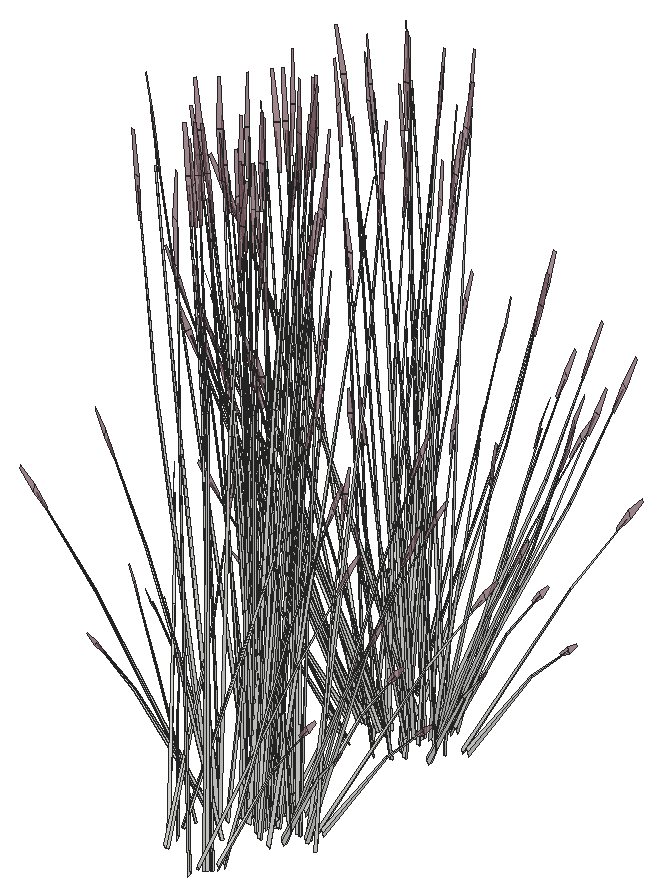
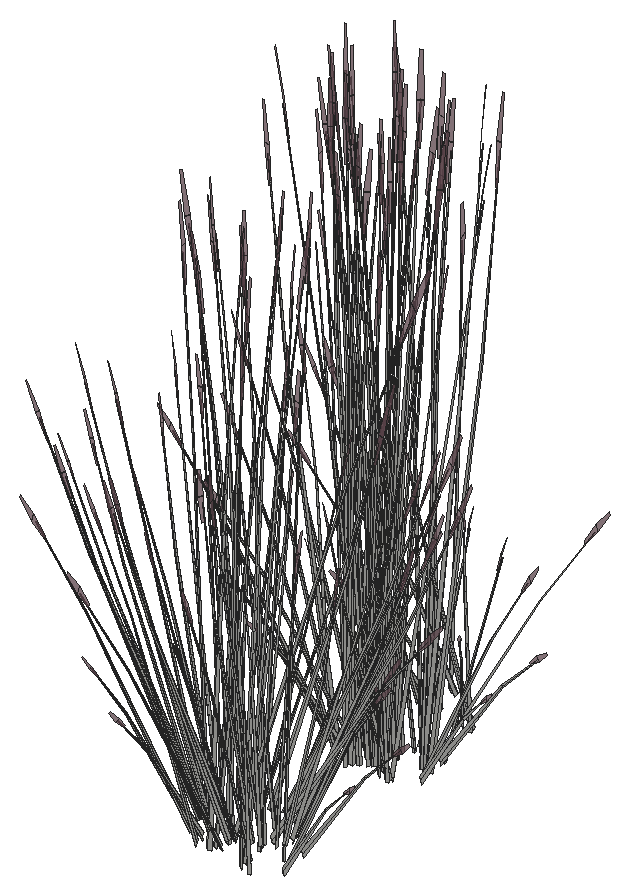
# SketchUp Ruby script. Lengths in inches.
U = 1.inch
M = Sketchup.active_model
def pt(a) = Geom::Point3d.new(a.map { |v| v * U })
def face(e, loops, mat)
  f = e.add_face(loops[0].map { |a| pt(a) })
  loops[1..].each { |l| e.add_face(l.map { |a| pt(a) }).erase! }
  f.material = f.back_material = mat if mat
  f
end
# faces: each face lists its corners as indices into pts; further lists are holes
def faces(e, pts, list, mat = nil) = list.each { |f| face(e, (f[0].is_a?(Array) ? f : [f]).map { |l| l.map { |i| pts[i] } }, mat) }
# xy, xz, yz: faces in a plane at the given z, y or x. An outline is a flat list of corners, or four numbers for a rectangle; further outlines are holes
def ring(l) = l.size == 4 ? [[l[0], l[1]], [l[2], l[1]], [l[2], l[3]], [l[0], l[3]]] : l.each_slice(2).to_a
def flat(e, list, mat, &to3) = list.each { |f| face(e, (f[0].is_a?(Array) ? f : [f]).map { |l| ring(l).map { |u, v| to3.(u, v) } }, mat) }
def xy(e, z, list, mat = nil) = flat(e, list, mat) { |x, y| [x, y, z] }
def xz(e, y, list, mat = nil) = flat(e, list, mat) { |x, z| [x, y, z] }
def yz(e, x, list, mat = nil) = flat(e, list, mat) { |y, z| [x, y, z] }
def lines(e, pts, list) = list.each { |a, b| e.add_line(pt(pts[a]), pt(pts[b])) }
# prism: a flat outline (further loops are holes) pulled along v
def prism(e, loops, v, mat = nil)
  f = face(e, loops, mat); d = Geom::Vector3d.new(v.map { |x| x * U })
  f.pushpull(f.normal.samedirection?(d) ? d.length : -d.length)
end
def box(e, o, s, mat = nil) = prism(e, [[o, [o[0] + s[0], o[1], o[2]], [o[0] + s[0], o[1] + s[1], o[2]], [o[0], o[1] + s[1], o[2]]]], [0, 0, s[2]], mat)
def at(x, y, z, deg = 0) = Geom::Transformation.translation(pt([x, y, z])) * Geom::Transformation.rotation(ORIGIN, Z_AXIS, deg.degrees)
def axes(o, x, y, z) = Geom::Transformation.new([*x, 0, *y, 0, *z, 0, *pt(o).to_a, 1])
def part(name) = M.definitions.add(name)
# library, detail: a bought-in or finely detailed component or shape, given as its bounding box
def library(name, o, s) = part(name).tap { |d| box(d.entities, o, s) }
def detail(e, o, s) = box(e.add_group.entities, o, s)
def put(e, d, t, mat = nil) = e.add_instance(d, t).tap { |i| i.material = mat if mat }
def group(e, t, mat = nil) = e.add_group.tap { |g| g.transformation = t; g.material = mat if mat }.entities
root = M.entities
M.materials.add("LightPink_Translucent").color = [144, 107, 117]
M.materials["LightPink_Translucent"].alpha = 0.75
c1 = part("blade")
p = [[2.15,0.21,22],[0,0.17,0],[0.09,0.45,0],[2.18,0.31,22],[2.29,0.31,22],[0.38,0.45,0],
  [2.48,0.24,33],[2.49,0.24,33],[2.48,0.22,33]]
faces(c1.entities,p,[[0,1,2,3],[4,5,2,3],[6,3,4,7],[8,0,3,6]])
c2 = part("seeds")
p = [[0.3,-0.1,1.38],[-0.01,-0.03,1.59],[-0.01,-0.03,0.03],[0.14,-0.07,-0.07],[0.29,-0.03,3],[0.15,0.01,3.11]]
faces(c2.entities,p,[[0,1,2,3],[1,0,4,5]],"LightPink_Translucent")
c3 = part("blade with seeds")
put(c3.entities,c1,at(0,0,0))
put(c3.entities,c2,axes([2.4,0.25,30.99],[1.5799,-0.05474,1.17369],[-0.12525,1.92788,0.29478],[-0.07173,-0.02425,1.56792]))
put(root,c3,axes([273.84,375.7,124.88],[1.11998,0.21207,0.30756],[-0.2802,0.75803,-0.36492],[-0.18537,0.09487,1.64885]))
put(root,c3,axes([275.27,375.64,125.3125],[-0.5037,-0.18761,1.1486],[0.6504,-0.19062,0.84392],[0.17543,0.16147,0.25299]))
put(root,c3,axes([274.52,376.11,124.92],[0.55932,0.6538,0],[-0.93577,0.36461,-0.51607],[-0.21313,0.08304,1.63711]))
put(root,c3,axes([274.04,373.52,125.39],[-0.02444,-0.61432,1.41272],[1.10603,0.15924,0.59816],[-0.26159,0.33615,1.3335]))
put(root,c3,axes([270.82,381.5,124.95],[-0.55932,-0.6538,0],[0.93577,-0.36461,-0.51607],[0.21313,-0.08304,1.63711]))
put(root,c3,axes([272.05,380.71,124.71],[-0.61821,0.37431,-0.03893],[-0.56645,-0.40995,-0.17649],[-0.03988,-0.11616,0.58215]))
put(root,c3,axes([275.35,376.49,125.22],[-0.57368,-0.02046,1.0506],[0.37886,-0.43461,0.58006],[0.22663,0.15441,0.8241]))
put(root,c3,axes([276.55,382.52,125.17],[-0.31959,-0.01933,1.43002],[-0.32741,-0.51843,-0.30754],[0.39262,-0.14666,0.61141]))
put(root,c3,axes([273.48,375.4375,125.14],[0.01579,-0.21629,1.43002],[0.75442,-0.24159,-0.30754],[0.23289,0.25887,0.61141]))
put(root,c3,axes([276.92,381.57,125.35],[-0.29798,0.33213,1.1486],[-0.25612,-0.44624,0.84392],[0.24611,-0.11182,0.25299]))
put(root,c3,axes([270.05,377.24,125.3125],[-0.02315,-0.38796,1.1486],[0.57853,0.27671,0.84392],[-0.11378,0.18492,0.25299]))
put(root,c3,axes([268.98,381.39,124.71],[-0.25807,0.53277,-0.03893],[-0.79428,-0.16389,-0.17649],[-0.1206,-0.08714,0.58215]))
put(root,c3,axes([269.57,376.4,125.37],[0.8127,-0.11554,0.06507],[0.18684,0.46549,-0.86304],[-0.05152,0.23564,0.7736]))
put(root,c3,axes([268.55,383.82,124.95],[-1.11865,0,0],[0,-0.72922,-0.51607],[0,-0.16609,1.63711]))
put(root,c3,axes([268.74,382.52,125.17],[0.17466,0.18165,1.43002],[-0.40248,0.49377,-0.30754],[-0.41327,-0.11802,0.61141]))
put(root,c3,axes([269.42,383.63,124.91],[-0.83213,0.54855,0.30756],[-0.83263,-0.54278,-0.36492],[-0.02906,-0.15578,1.64885]))
put(root,c3,axes([271.85,376.06,127.53],[0.42698,0.53052,-0.71045],[-0.87893,0.29566,0.08574],[0.09984,0.25633,1.00501]))
put(root,c3,axes([269.38,376.89,125.14],[0.28231,-0.10293,1.43002],[0.69701,0.31035,-0.30754],[-0.20746,0.26854,0.61141]))
put(root,c3,axes([272.0625,383.88,125.01],[1.00799,0.31623,0.24065],[-0.48511,0.65709,0.50002],[0,-0.15147,1.60543]))
put(root,c3,axes([267.7,383.0625,125.35],[0.57115,-0.04669,1.1486],[-0.36229,0.41137,0.84392],[-0.28224,-0.06171,0.25299]))
put(root,c3,axes([271.74,383.44,125.3],[-0.97146,0.04028,0.44739],[-0.08785,-0.66859,-0.21531],[0.17391,-0.06776,1.43643]))
put(root,c3,axes([269.23,383.93,125.06],[0,0.65246,0.49651],[-1.00089,0,0],[0,-0.1486,1.57504]))
put(root,c3,axes([274.94,381.66,124.96],[0.55932,-0.6538,0],[0.93577,0.36461,-0.51607],[0.21313,0.08304,1.63711]))
put(root,c3,axes([271.7,383.68,124.94],[0.38895,0.72959,0.45755],[-1.11135,0.2537,0.17955],[0.01358,-0.13406,1.58856]))
put(root,c3,axes([277.14,384.24,124.5625],[-0.57619,0.0783,1.41583],[-0.09171,-0.62326,0.08104],[0.40356,-0.09434,0.80566]))
put(root,c3,axes([278.19,383.69,124.84],[-0.55463,-0.41721,-0.06488],[0.60744,-0.38228,-0.29416],[0.17212,-0.02691,0.97024]))
put(root,c3,axes([271.51,384.26,125.3],[-0.43405,0.58792,0.44739],[-0.90188,-0.28295,-0.21531],[0,-0.13553,1.43643]))
put(root,c3,axes([273.1,383.75,124.79],[0,-0.75495,0],[1.11865,0,0],[0,0,1.79456]))
put(root,c3,axes([274.46,382,125.06],[-0.83726,-0.32623,0.49651],[0.50045,-0.58498,0],[0.19069,0.0743,1.57504]))
put(root,c3,axes([272.57,383.27,124.94],[-0.74176,0.59212,0.45755],[-0.88124,-0.52269,0.17955],[0.17882,-0.05909,1.58856]))
put(root,c3,axes([273.38,384.33,124.88],[-0.83213,-0.56158,-0.06131],[0.83263,-0.56193,0],[-0.02906,-0.01961,1.75571]))
put(root,c3,axes([271.29,382.3,125.05],[-0.25843,0.64844,0.17642],[-0.9457,-0.1835,0.35086],[0.16336,-0.00316,1.60407]))
put(root,c3,axes([273.26,383.02,125.2],[0.17258,-0.58229,0.1448],[0.84319,0.10108,-0.41347],[0.15345,0.05979,1.26744]))
put(root,c3,axes([271.8,384.4,124.94],[1.13071,0.13747,0.45755],[-0.23011,0.77639,0.17955],[-0.16524,-0.07497,1.58856]))
put(root,c3,axes([272.9,383.17,125.3],[-0.53742,-0.54764,0.44739],[0.81403,-0.38564,-0.21531],[0.17391,0.06776,1.43643]))
put(root,c3,axes([271.19,385.64,125.05],[0.96132,-0.17317,0.17642],[0.23737,0.64447,0.35086],[-0.08574,-0.0939,1.60407]))
put(root,c3,axes([273.86,383.92,124.79],[1.00089,0,0],[0,0.67548,0],[0,0,1.78407]))
put(root,c3,axes([274.15,382.33,125.05],[-0.96132,0.17317,0.17642],[-0.23737,-0.64447,0.35086],[0.08574,0.0939,1.60407]))
put(root,c3,axes([273.54,383.57,124.96],[-1.13071,-0.13747,0.49198],[0.23011,-0.77639,0.19306],[0.16524,0.07497,1.70813]))
put(root,c3,axes([272.64,385.49,124.78],[-0.29189,-0.56252,0],[0.83351,-0.19699,0],[0,0,1.54371]))
put(root,c3,axes([272.08,384.95,125.2],[-0.17258,0.58229,0.1448],[-0.84319,-0.10108,-0.41347],[-0.15345,-0.05979,1.26744]))
put(root,c3,axes([274.05,385.68,125.05],[0.25843,-0.64844,0.17642],[0.9457,0.1835,0.35086],[-0.16336,0.00316,1.60407]))
put(root,c3,axes([273.84,384.2,124.8],[0.62448,0.42144,0],[-0.62448,0.42144,0],[0,0,1.69266]))
put(root,c3,axes([275.53,384.02,125.05],[-0.70288,-0.47526,0.17642],[0.70832,-0.46097,0.35086],[-0.07763,0.09706,1.60407]))
put(root,c3,axes([278.34,384.46,125.35],[-0.55274,0.10771,1.1486],[0.26018,-0.44517,0.84392],[0.29323,0.03046,0.25299]))
put(root,c3,axes([272.43,385.74,124.78],[-0.90188,-0.29293,0],[0.43405,-0.60866,0],[0,0,1.62707]))
put(root,c3,axes([270.88,385.97,125.06],[0.83726,0.32623,0.49651],[-0.50045,0.58498,0],[-0.19069,-0.0743,1.57504]))
put(root,c3,axes([273.83,383.71,125.3],[0.43405,-0.58792,0.44739],[0.90188,0.28295,-0.21531],[0,0.13553,1.43643]))
put(root,c3,axes([273.67,384.05,124.87],[0,0.75458,-0.05637],[-1.11865,0,0],[0,0.02371,1.79368]))
put(root,c3,axes([270.4,386.31,124.95],[-0.55932,0.6538,0],[-0.93577,-0.36461,-0.51607],[-0.21313,-0.08304,1.63711]))
put(root,c3,axes([276.11,384.04,125.06],[0,-0.65246,0.49651],[1.00089,0,0],[0,0.1486,1.57504]))
put(root,c3,axes([273.6,384.53,125.3],[0.97146,-0.04028,0.44739],[0.08785,0.66859,-0.21531],[-0.17391,0.06776,1.43643]))
put(root,c3,axes([274.21,383.85,125.2],[0.83351,-0.19028,0.1448],[0.29189,0.54335,-0.41347],[0,0.11958,1.26744]))
put(root,c3,axes([277.31,385.17,125.17],[-0.21545,-0.16047,1.43002],[0.28033,-0.53085,-0.30754],[0.43591,0.07191,0.61141]))
put(root,c3,axes([273.45,385.75,124.78],[0.90188,0.29293,0],[-0.43405,0.60866,0],[0,0,1.74954]))
put(root,c3,axes([273.8125,386.4,124.77],[-0.55235,-0.65609,-0.05142],[0.93577,-0.36461,0.51607],[-0.23059,0.06247,1.6363]))
put(root,c3,axes([273.62,384.81,125.2],[0.66093,0.39201,0.1448],[-0.5513,0.44227,-0.41347],[-0.15345,0.05979,1.26744]))
put(root,c3,axes([274.32,386.02,125.06],[0.83726,-0.32623,0.49651],[0.50045,0.58498,0],[-0.19069,0.0743,1.57504]))
put(root,c3,axes([273.13,385.51,124.87],[0.38895,0.74956,-0.06012],[-1.11135,0.26265,0],[0.01358,0.02618,1.72173]))
put(root,c3,axes([267.54,385.17,125.17],[0.3109,0.05356,1.43002],[0.20038,0.54709,-0.30754],[-0.42231,0.10241,0.61141]))
put(root,c3,axes([276.79,384.15,124.96],[1.11865,0,0],[0,0.72922,-0.51607],[0,0.16609,1.63711]))
put(root,c3,axes([276.34,384.52,124.78],[-1.1181,-0.00522,-0.04976],[0,-0.72922,0.49943],[-0.03514,0.166,1.58352]))
put(root,c3,axes([266.89,386.3125,125.35],[0.37283,-0.29571,1.1486],[0.14711,0.46813,0.84392],[-0.26943,0.08382,0.25299]))
put(root,c3,axes([273.84,386.06,124.91],[1.11998,0.21207,0.30756],[-0.2802,0.75803,-0.36492],[-0.18537,0.09487,1.64885]))
put(root,c3,axes([275.27,386,125.35],[-0.5037,-0.18761,1.1486],[0.6504,-0.19062,0.84392],[0.17543,0.16147,0.25299]))
put(root,c3,axes([274.52,386.48,124.95],[0.55932,0.6538,0],[-0.93577,0.36461,-0.51607],[-0.21313,0.08304,1.63711]))
put(root,c3,axes([274.04,383.89,125.42],[-0.02444,-0.61432,1.41272],[1.10603,0.15924,0.59816],[-0.26159,0.33615,1.3335]))
put(root,c3,axes([275.35,386.85,125.25],[-0.57368,-0.02046,1.0506],[0.37886,-0.43461,0.58006],[0.22663,0.15441,0.8241]))
put(root,c3,axes([273.48,385.8,125.17],[0.01579,-0.21629,1.43002],[0.75442,-0.24159,-0.30754],[0.23289,0.25887,0.61141]))
put(root,c3,axes([270.05,387.6,125.35],[-0.02315,-0.38796,1.1486],[0.57853,0.27671,0.84392],[-0.11378,0.18492,0.25299]))
put(root,c3,axes([269.57,386.76,125.4],[0.8127,-0.11554,0.06507],[0.18684,0.46549,-0.86304],[-0.05152,0.23564,0.7736]))
put(root,c3,axes([269.38,387.26,125.17],[0.28231,-0.10293,1.43002],[0.69701,0.31035,-0.30754],[-0.20746,0.26854,0.61141]))
put(root,c3,axes([274.1,398.08,124.51],[-0.25429,0.13207,1.43002],[-0.76157,-0.23115,-0.30754],[0.14117,-0.28747,0.61141]))
put(root,c3,axes([272.94,398.54,126.9],[-0.42698,-0.53052,-0.71045],[0.87893,-0.29566,0.08574],[-0.09984,-0.25633,1.00501]))
put(root,c3,axes([270.16,397.83,124.51],[-0.05417,0.21344,1.43002],[-0.79196,0.17867,-0.30754],[-0.18512,-0.27588,0.61141]))
put(root,c3,axes([274.72,399.06,126.9],[0.02328,-0.60353,-0.71045],[0.98022,0.04053,0.08574],[0.10344,-0.25568,1.00501]))
put(root,c3,axes([273.02,398.09,126.44],[0.2697,-0.50175,-0.35414],[0.78684,0.14635,0.4572],[-0.07215,-0.20201,0.87481]))
put(root,c3,axes([272.62,398.43,126.6],[-0.87941,-0.16356,-0.51099],[0.30143,-0.56078,-0.3958],[-0.08064,-0.22578,0.97773]))
put(root,c3,axes([273.16,397.03,124.68],[0.11476,0.38047,1.1486],[-0.63664,-0.21072,0.84392],[0.06851,-0.19481,0.25299]))
put(root,c3,axes([274.52,398.86,126.6],[-0.64041,-0.4384,-0.51099],[0.67652,-0.38394,-0.3958],[0.09744,-0.22274,0.97773]))
put(root,c3,axes([275.12,398.69,126.44],[0.60531,-0.34352,-0.35414],[0.573,0.39225,0.4572],[0.08718,-0.19929,0.87481]))
put(root,c3,axes([269.89,397.48,124.68],[0.46666,0.22709,1.1486],[-0.67962,0.13651,0.84392],[-0.14541,-0.17452,0.25299]))
put(root,c3,axes([271.02,398.6875,126.9],[-0.76283,-0.31537,-0.71045],[0.54213,-0.55263,0.08574],[-0.27638,-0.1883,1.00501]))
put(root,c3,axes([270.75,398.27,126.44],[-0.13817,-0.52554,-0.35414],[0.78985,-0.13877,0.4572],[-0.21215,-0.1506,0.87481]))
put(root,c3,axes([270.66,398.7,126.6],[-0.88277,0.1551,-0.51099],[-0.15442,-0.58737,-0.3958],[-0.23711,-0.16832,0.97773]))
put(root,c3,axes([275.875,400.11,126.9],[0.4673,-0.51481,-0.71045],[0.81887,0.36587,0.08574],[0.27902,-0.18652,1.00501]))
put(root,c3,axes([275.85,399.87,126.6],[-0.22982,-0.59576,-0.51099],[0.87033,-0.10422,-0.3958],[0.24941,-0.16002,0.97773]))
put(root,c3,axes([272.84,402.26,125.24],[0.77308,0.2631,1.51261],[-0.75736,0.56681,0.59816],[-0.33924,-0.33594,1.26806]))
put(root,c3,axes([276.55,399.63,124.51],[-0.31959,-0.01933,1.43002],[-0.32741,-0.51843,-0.30754],[0.39262,-0.14666,0.61141]))
put(root,c3,axes([276.92,398.68,124.68],[-0.29798,0.33213,1.1486],[-0.25612,-0.44624,0.84392],[0.24611,-0.11182,0.25299]))
put(root,c3,axes([276.49,399.93,126.44],[0.77872,-0.09325,-0.35414],[0.20563,0.53305,0.4572],[0.22316,-0.14318,0.87481]))
put(root,c3,axes([268.92,399.2,126.44],[-0.50902,-0.40851,-0.35414],[0.58122,-0.38671,0.4572],[-0.29531,-0.05884,0.87481]))
put(root,c3,axes([269.46,399.47,126.9],[-0.89428,-0.01571,-0.71045],[0.06006,-0.66153,0.08574],[-0.37886,-0.06981,1.00501]))
put(root,c3,axes([269.17,399.6,126.6],[-0.6496,0.4322,-0.51099],[-0.5689,-0.45657,-0.3958],[-0.33005,-0.06576,0.97773]))
put(root,c3,axes([267.7,400.18,124.68],[0.57115,-0.04669,1.1486],[-0.36229,0.41137,0.84392],[-0.28224,-0.06171,0.25299]))
put(root,c3,axes([271.74,400.56,124.63],[-0.97146,0.04028,0.44739],[-0.08785,-0.66859,-0.21531],[0.17391,-0.06776,1.43643]))
put(root,c3,axes([269.23,401.04,124.39],[0,0.65246,0.49651],[-1.00089,0,0],[0,-0.1486,1.57504]))
put(root,c3,axes([276.26,401.1875,126.6],[0.24236,-0.59349,-0.51099],[0.83094,0.20343,-0.3958],[0.33455,-0.05442,0.97773]))
put(root,c3,axes([271.51,401.37,124.63],[-0.43405,0.58792,0.44739],[-0.90188,-0.28295,-0.21531],[0,-0.13553,1.43643]))
put(root,c3,axes([274.46,399.11,124.39],[-0.83726,-0.32623,0.49651],[0.50045,-0.58498,0],[0.19069,0.0743,1.57504]))
put(root,c3,axes([276.1,401.4,126.9],[0.78611,-0.28816,-0.71045],[0.4381,0.59317,0.08574],[0.37982,-0.06738,1.00501]))
put(root,c3,axes([271.29,399.41,124.39],[-0.25843,0.64844,0.17642],[-0.9457,-0.1835,0.35086],[0.16336,-0.00316,1.60407]))
put(root,c3,axes([272.9,400.28,124.63],[-0.53742,-0.54764,0.44739],[0.81403,-0.38564,-0.21531],[0.17391,0.06776,1.43643]))
put(root,c3,axes([271.19,402.75,124.39],[0.96132,-0.17317,0.17642],[0.23737,0.64447,0.35086],[-0.08574,-0.0939,1.60407]))
put(root,c3,axes([276.76,401.46,126.44],[0.74348,0.18202,-0.35414],[-0.21685,0.53102,0.4572],[0.29933,-0.04869,0.87481]))
put(root,c3,axes([268.03,400.61,126.44],[-0.74348,-0.18202,-0.35414],[0.21685,-0.53102,0.4572],[-0.29933,0.04869,0.87481]))
put(root,c3,axes([274.15,399.44,124.39],[-0.96132,0.17317,0.17642],[-0.23737,-0.64447,0.35086],[0.08574,0.0939,1.60407]))
put(root,c3,axes([274.05,402.79,124.39],[0.25843,-0.64844,0.17642],[0.9457,0.1835,0.35086],[-0.16336,0.00316,1.60407]))
put(root,c3,axes([270.29,400.53,125.26],[0.25429,-0.09438,1.77064],[0.08769,0.65901,0.13857],[-0.5508,0.08745,0.63284]))
put(root,c3,axes([275.53,401.13,124.39],[-0.70288,-0.47526,0.17642],[0.70832,-0.46097,0.35086],[-0.07763,0.09706,1.60407]))
put(root,c3,axes([278.34,401.57,124.68],[-0.55274,0.10771,1.1486],[0.26018,-0.44517,0.84392],[0.29323,0.03046,0.25299]))
put(root,c3,axes([270.88,403.08,124.39],[0.83726,0.32623,0.49651],[-0.50045,0.58498,0],[-0.19069,-0.0743,1.57504]))
put(root,c3,axes([273.83,400.82,124.63],[0.43405,-0.58792,0.44739],[0.90188,0.28295,-0.21531],[0,0.13553,1.43643]))
put(root,c3,axes([268.54,400.88,126.6],[-0.24236,0.59349,-0.51099],[-0.83094,-0.20343,-0.3958],[-0.33455,0.05442,0.97773]))
put(root,c3,axes([276.11,401.15,124.39],[0,-0.65246,0.49651],[1.00089,0,0],[0,0.1486,1.57504]))
put(root,c3,axes([273.6,401.64,124.63],[0.97146,-0.04028,0.44739],[0.08785,0.66859,-0.21531],[-0.17391,0.06776,1.43643]))
put(root,c3,axes([277.31,402.28,124.51],[-0.21545,-0.16047,1.43002],[0.28033,-0.53085,-0.30754],[0.43591,0.07191,0.61141]))
put(root,c3,axes([275.33,402.6,126.9],[0.89428,0.01571,-0.71045],[-0.06006,0.66153,0.08574],[0.37886,0.06981,1.00501]))
put(root,c3,axes([274.32,403.13,124.39],[0.83726,-0.32623,0.49651],[0.50045,0.58498,0],[-0.19069,0.0743,1.57504]))
put(root,c3,axes([267.54,402.28,124.51],[0.3109,0.05356,1.43002],[0.20038,0.54709,-0.30754],[-0.42231,0.10241,0.61141]))
put(root,c3,axes([266.89,403.42,124.68],[0.37283,-0.29571,1.1486],[0.14711,0.46813,0.84392],[-0.26943,0.08382,0.25299]))
put(root,c3,axes([275.87,402.88,126.44],[0.50902,0.40851,-0.35414],[-0.58122,0.38671,0.4572],[0.29531,0.05884,0.87481]))
put(root,c3,axes([268.3,402.14,126.44],[-0.77872,0.09325,-0.35414],[-0.20563,-0.53305,0.4572],[-0.22316,0.14318,0.87481]))
put(root,c3,axes([275.27,403.11,124.68],[-0.5037,-0.18761,1.1486],[0.6504,-0.19062,0.84392],[0.17543,0.16147,0.25299]))
put(root,c3,axes([268.94,402.21,126.6],[0.22982,0.59576,-0.51099],[-0.87033,0.10422,-0.3958],[-0.24941,0.16002,0.97773]))
put(root,c3,axes([274.04,401,124.76],[-0.02444,-0.61432,1.41272],[1.10603,0.15924,0.59816],[-0.26159,0.33615,1.3335]))
put(root,c3,axes([274.13,403.37,126.6],[0.88277,-0.1551,-0.51099],[0.15442,0.58737,-0.3958],[0.23711,0.16832,0.97773]))
put(root,c3,axes([275.35,403.96,124.58],[-0.57368,-0.02046,1.0506],[0.37886,-0.43461,0.58006],[0.22663,0.15441,0.8241]))
put(root,c3,axes([273.48,402.91,124.51],[0.01579,-0.21629,1.43002],[0.75442,-0.24159,-0.30754],[0.23289,0.25887,0.61141]))
put(root,c3,axes([269.67,403.38,126.44],[-0.60531,0.34352,-0.35414],[-0.573,-0.39225,0.4572],[-0.08718,0.19929,0.87481]))
put(root,c3,axes([270.05,404.71,124.68],[-0.02315,-0.38796,1.1486],[0.57853,0.27671,0.84392],[-0.11378,0.18492,0.25299]))
put(root,c3,axes([270.27,403.22,126.92],[0.64041,0.4384,-0.5672],[-0.67652,0.38394,-0.43934],[-0.09744,0.22274,1.08528]))
put(root,c3,axes([272.17,403.64,126.6],[0.87941,0.16356,-0.51099],[-0.30143,0.56078,-0.3958],[0.08064,0.22578,0.97773]))
put(root,c3,axes([271.77,403.99,126.44],[-0.2697,0.50175,-0.35414],[-0.78684,-0.14635,0.4572],[0.07215,0.20201,0.87481]))
put(root,c3,axes([270.07,403.02,127.25],[-0.02328,0.60353,-0.7886],[-0.98022,-0.04053,0.09517],[-0.10344,0.25568,1.11556]))
put(root,c3,axes([271.85,403.53,126.9],[0.42698,0.53052,-0.71045],[-0.87893,0.29566,0.08574],[0.09984,0.25633,1.00501]))
put(root,c3,axes([269.38,404.37,124.51],[0.28231,-0.10293,1.43002],[0.69701,0.31035,-0.30754],[-0.20746,0.26854,0.61141]))
put(root,c3,axes([269.74,403.87,125.28],[0.01966,-0.33682,1.54345],[0.88405,0.17791,0.21329],[-0.0766,0.35897,0.72882]))
